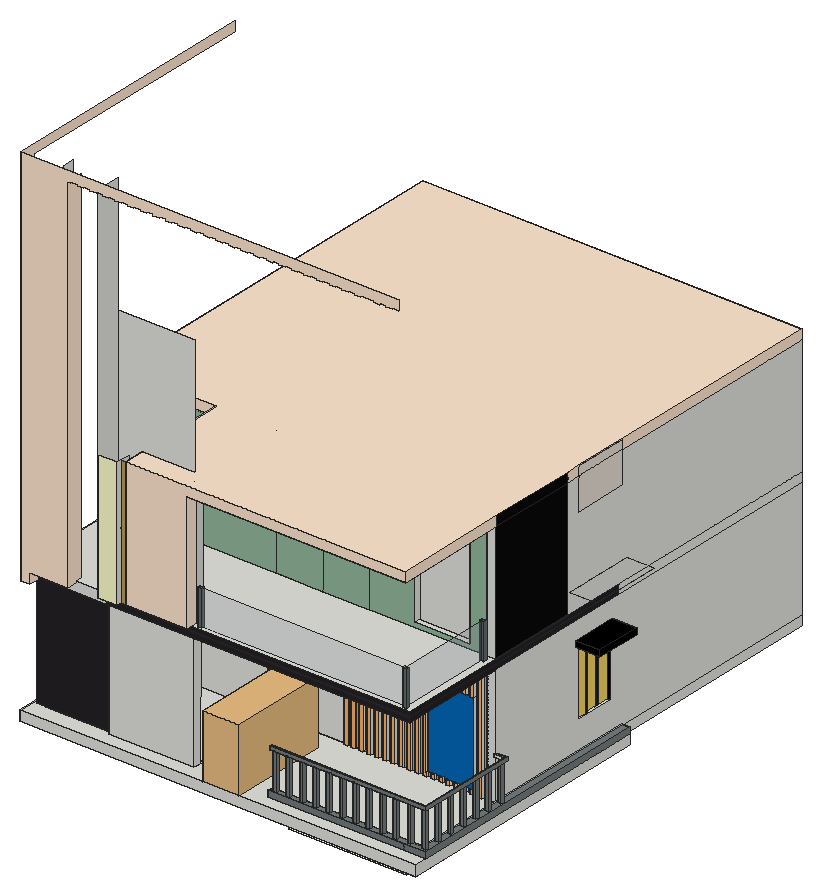
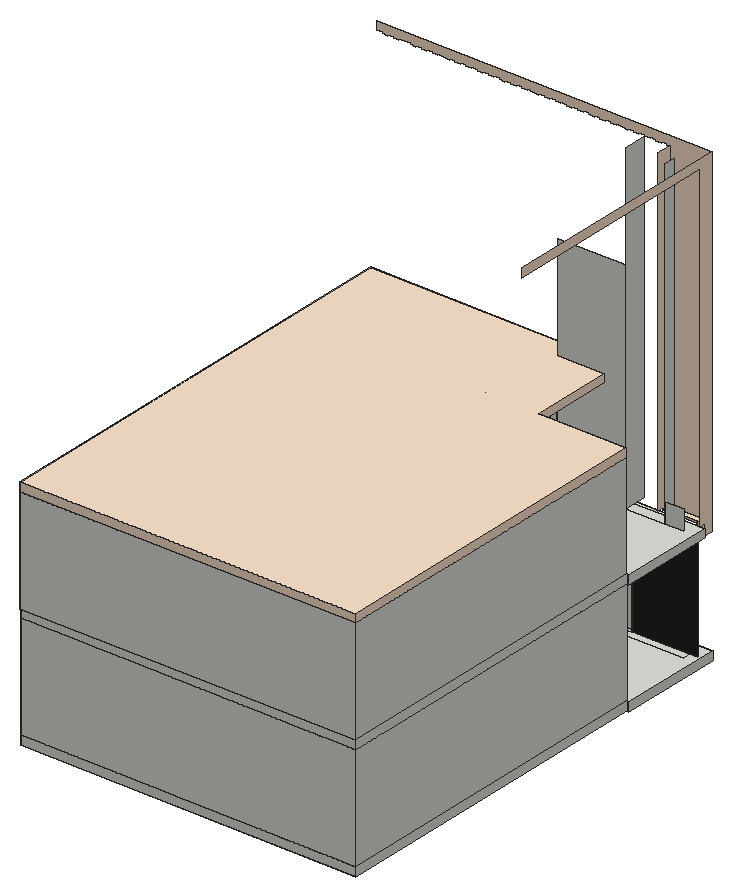
# SketchUp Ruby script. Lengths in inches.
U = 1.inch
M = Sketchup.active_model
def pt(a) = Geom::Point3d.new(a.map { |v| v * U })
def face(e, loops, mat)
  f = e.add_face(loops[0].map { |a| pt(a) })
  loops[1..].each { |l| e.add_face(l.map { |a| pt(a) }).erase! }
  f.material = f.back_material = mat if mat
  f
end
# faces: each face lists its corners as indices into pts; further lists are holes
def faces(e, pts, list, mat = nil) = list.each { |f| face(e, (f[0].is_a?(Array) ? f : [f]).map { |l| l.map { |i| pts[i] } }, mat) }
# xy, xz, yz: faces in a plane at the given z, y or x. An outline is a flat list of corners, or four numbers for a rectangle; further outlines are holes
def ring(l) = l.size == 4 ? [[l[0], l[1]], [l[2], l[1]], [l[2], l[3]], [l[0], l[3]]] : l.each_slice(2).to_a
def flat(e, list, mat, &to3) = list.each { |f| face(e, (f[0].is_a?(Array) ? f : [f]).map { |l| ring(l).map { |u, v| to3.(u, v) } }, mat) }
def xy(e, z, list, mat = nil) = flat(e, list, mat) { |x, y| [x, y, z] }
def xz(e, y, list, mat = nil) = flat(e, list, mat) { |x, z| [x, y, z] }
def yz(e, x, list, mat = nil) = flat(e, list, mat) { |y, z| [x, y, z] }
def lines(e, pts, list) = list.each { |a, b| e.add_line(pt(pts[a]), pt(pts[b])) }
# prism: a flat outline (further loops are holes) pulled along v
def prism(e, loops, v, mat = nil)
  f = face(e, loops, mat); d = Geom::Vector3d.new(v.map { |x| x * U })
  f.pushpull(f.normal.samedirection?(d) ? d.length : -d.length)
end
def box(e, o, s, mat = nil) = prism(e, [[o, [o[0] + s[0], o[1], o[2]], [o[0] + s[0], o[1] + s[1], o[2]], [o[0], o[1] + s[1], o[2]]]], [0, 0, s[2]], mat)
def at(x, y, z, deg = 0) = Geom::Transformation.translation(pt([x, y, z])) * Geom::Transformation.rotation(ORIGIN, Z_AXIS, deg.degrees)
def axes(o, x, y, z) = Geom::Transformation.new([*x, 0, *y, 0, *z, 0, *pt(o).to_a, 1])
def part(name) = M.definitions.add(name)
# library, detail: a bought-in or finely detailed component or shape, given as its bounding box
def library(name, o, s) = part(name).tap { |d| box(d.entities, o, s) }
def detail(e, o, s) = box(e.add_group.entities, o, s)
def put(e, d, t, mat = nil) = e.add_instance(d, t).tap { |i| i.material = mat if mat }
def group(e, t, mat = nil) = e.add_group.tap { |g| g.transformation = t; g.material = mat if mat }.entities
root = M.entities
M.materials.add("C01_Vanilla_Cream").color = [255, 230, 206]
M.materials.add("C03_Honey_Glow").color = [255, 178, 101]
M.materials.add("C04_Amber_Sunshine").color = [255, 152, 49]
M.materials.add("C05_Golden_Blaze").color = [255, 123, 0]
M.materials.add("E01_Mint_Frost").color = [255, 255, 204]
M.materials.add("Glass_Basic_01").color = [161, 173, 186]
M.materials["Glass_Basic_01"].alpha = 0.25
M.materials.add("Glass_Mirror_01").color = [4, 105, 185]
M.materials.add("Glass_Mirror_2").color = [185, 158, 90]
M.materials.add("Glass_Mirror_3").color = [244, 212, 100]
M.materials.add("Glass_Mirror_4").color = [147, 185, 156]
M.materials.add("GreyOffset").color = [97, 108, 109]
M.materials.add("M08_Obsidian_Black1").color = [30, 30, 30]
M.materials.add("M09_Shadow_Night").color = [0, 0, 0]
M.materials.add("Marble_01_1K").color = [230, 221, 211]
M.materials.add("Marble_07_1K").color = [36, 34, 36]
M.materials.add("Metal_32_1K").color = [117, 124, 125]
M.materials.add("NERO MARQUINA 02").color = [10, 10, 10]
M.materials.add("[Color_000]").color = [255, 255, 255]
c1 = part("Group\#12")
xy(c1.entities,36,[[0,0,3.82,2.79]],"Metal_32_1K")
xz(c1.entities,0,[[0,0,3.82,36]],"Metal_32_1K")
xz(c1.entities,2.79,[[0,0,3.82,36]],"Metal_32_1K")
yz(c1.entities,0,[[0,0,2.79,36]],"Metal_32_1K")
yz(c1.entities,3.82,[[0,0,2.79,36]],"Metal_32_1K")
c2 = part("Group\#11")
xy(c2.entities,36,[[0,0,3.82,2.79]],"Metal_32_1K")
xz(c2.entities,0,[[0,0,3.82,36]],"Metal_32_1K")
xz(c2.entities,2.79,[[0,0,3.82,36]],"Metal_32_1K")
yz(c2.entities,0,[[0,0,2.79,36]],"Metal_32_1K")
yz(c2.entities,3.82,[[0,0,2.79,36]],"Metal_32_1K")
c3 = library("Group_2",[-1.28,-0.39,0],[21.22,20.51,48.44])
xy(root,97.49,[[307.1875,182.1,366.58,186.51],[366.83,182.1,426.21,186.22]],"[Color_000]")
xy(root,120,[[60.23,165,180,171],[222,171,287.05,179.92],[222,179.92,287.05,180],[222,180,287.05,204.3],[435.75,196.73,444.75,197.01,444,220.51,444,273,435,273,435,220.22]])
xy(root,130,[[135.41,168,222,171],[69,171,222,179.92]])
xy(root,249.85,[[60,151,69,161]],"C01_Vanilla_Cream")
xy(root,259.85,[[135.55,154,155.45,168],[89.98,168,135.55,180]])
xy(root,259.85,[[69,151,107.56,161]],"C01_Vanilla_Cream")
xz(root,151,[[60,249.85,69,249.85,69,259.85,107.56,259.85,107.56,628.54,111.09,628.54,111.09,629.54,117.48,629.54,117.48,628.54,123.87,628.54,123.87,629.54,130.25,629.54,130.25,628.54,136.64,628.54,136.64,629.54,143.03,629.54,143.03,628.54,149.41,628.54,149.41,629.54,155.8,629.54,155.8,628.54,162.1875,628.54,162.1875,629.54,168.57,629.54,168.57,628.54,174.96,628.54,174.96,629.54,181.35,629.54,181.35,628.54,187.73,628.54,187.73,629.54,194.12,629.54,194.12,628.54,200.51,628.54,200.51,629.54,206.89,629.54,206.89,628.54,213.28,628.54,213.28,629.54,219.67,629.54,219.67,628.54,226.05,628.54,226.05,629.54,232.4375,629.54,232.4375,628.54,238.83,628.54,238.83,629.54,245.21,629.54,245.21,628.54,251.6,628.54,251.6,629.54,257.98,629.54,257.98,628.54,264.37,628.54,264.37,629.54,270.76,629.54,270.76,628.54,277.14,628.54,277.14,629.54,283.53,629.54,283.53,628.54,289.92,628.54,289.92,629.54,296.3,629.54,296.3,628.54,302.69,628.54,302.69,629.54,309.08,629.54,309.08,628.54,315.46,628.54,315.46,629.54,321.85,629.54,321.85,628.54,328.24,628.54,328.24,629.54,334.625,629.54,334.625,628.54,341.01,628.54,341.01,629.54,347.4,629.54,347.4,628.54,353.78,628.54,353.78,629.54,360.17,629.54,360.17,628.54,366.56,628.54,366.56,629.54,372.94,629.54,372.94,628.54,379.33,628.54,379.33,629.54,385.72,629.54,385.72,628.54,392.1,628.54,392.1,629.54,398.49,629.54,398.49,628.54,404.88,628.54,404.88,629.54,417.65,629.54,417.65,628.54,424.04,628.54,424.04,629.54,430.42,629.54,430.42,628.54,436.81,628.54,436.81,629.54,443.2,629.54,443.2,639.54,60,639.54]],"C01_Vanilla_Cream")
xz(root,154,[[135.55,259.85,155.45,389.69]],"E01_Mint_Frost")
xz(root,159,[[155.45,259.85,160.13,389.69]],"Glass_Mirror_2")
xz(root,161,[[60,249.85,69,261.88],[69,259.85,107.56,261.88]],"C01_Vanilla_Cream")
xz(root,168,[[135.41,130,222,249.85]])
xz(root,168.1,[[230.8,259.85,434.6,295.85]],"Glass_Basic_01")
xz(root,171,[[60,130,135.41,249.85]],"Marble_07_1K")
xz(root,180,[[69,259.85,89.98,282.89],[135.55,259.85,213,509.54]])
yz(root,60,[[151,249.85,151,639.54,422.07,639.54,422.07,629.54,168,629.54,168,261.88,161,261.88,161,249.85]],"C01_Vanilla_Cream")
yz(root,69,[[151,249.85,161,259.85]],"C01_Vanilla_Cream")
yz(root,89.98,[[168,259.85,180,629.54]])
yz(root,107.56,[[151,259.85,161,259.85,161,261.88,168,261.88,168,628.54,151,628.54]],"C01_Vanilla_Cream")
yz(root,135.41,[[168,130,171,249.85]])
yz(root,135.55,[[154,259.85,180,629.54]])
yz(root,155.45,[[154,259.85,159,389.69],[159,259.85,168,389.69]])
yz(root,222,[[168,130,175.46,130,176.59,249.8,176.59,249.85,168,249.85]])
yz(root,436.72,[[169.55,259.85,264.51,295.85]],"Glass_Basic_01")
p = [[222.23,171,379.69],[222.23,171,259.85],[221.39,180,259.85],[221.39,180,379.69],[222,168,249.85],[222,168,389.69],
  [444,363.42,259.85],[444,273.3,259.85],[213,180,259.85]]
faces(root,p,[[0,1,2,3]])
lines(root,p,[[4,5],[6,7],[8,2]])
g1 = group(root,at(60,273,120))
xy(g1,0,[[-3,-119.23,-3,0,0,0,0,387,384,387,384,152.46,397.91,152.46,397.91,-119.23]])
xy(g1,10,[[-3,-119.23,397.91,-119.23,397.91,-105.79,237.85,-105.79,237.85,-100,389.74,-100,389.74,152.46,384,152.46,384,387,0,387,0,0,-3,0],[237.85,-105.79,397.91,-105.79,397.91,152.46,389.74,152.46,389.74,-100,237.85,-100]])
xy(g1,16,[[237.85,-105.79,397.91,-105.79,397.91,152.46,389.74,152.46,389.74,-100,237.85,-100]],"Metal_32_1K")
xy(g1,52,[[237.68,-103.375,237.68,-101.59,378.28,-101.59,378.28,-101.48,393.9,-101.48,393.9,-2.71,384,-2.71,384,0,395.84,0,395.84,-103.375]])
xy(g1,55,[[237.68,-103.375,395.84,-103.375,395.84,0,384,0,384,-2.71,393.9,-2.71,393.9,-101.48,378.28,-101.48,378.28,-101.59,237.68,-101.59]],"Metal_32_1K")
xz(g1,-119.23,[[-3,0,397.91,10]])
xz(g1,-105.79,[[237.85,10,375,16],[375,10,397.91,16]],"Metal_32_1K")
xz(g1,-103.375,[[237.68,52,395.84,55]],"Metal_32_1K")
xz(g1,-101.59,[[237.68,52,378.28,55]],"Metal_32_1K")
xz(g1,-101.48,[[378.28,52,393.9,55]])
xz(g1,-100,[[237.85,10,375,16],[375,10,389.74,16]])
xz(g1,-2.71,[[384,52,393.9,55]])
xz(g1,0,[[-3,0,0,10],[384,52,395.84,55]])
xz(g1,152.46,[[384,0,397.91,9.85],[384,9.85,397.91,10],[389.74,10,397.91,16]])
xz(g1,387,[[0,0,384,10]])
yz(g1,-3,[[-119.23,0,0,10]])
yz(g1,0,[[0,0,387,10]])
yz(g1,237.68,[[-103.375,52,-101.59,55]],"Metal_32_1K")
yz(g1,237.85,[[-105.79,10,-100,16]],"Metal_32_1K")
yz(g1,378.28,[[-101.59,52,-101.48,55]])
yz(g1,384,[[152.46,0,387,10],[-2.71,52,0,55]])
yz(g1,389.74,[[-100,10,152.46,16]])
yz(g1,393.9,[[-101.48,52,-2.71,55]])
yz(g1,395.84,[[-103.375,52,0,55]],"Metal_32_1K")
yz(g1,397.91,[[-119.23,0,152.46,10]])
yz(g1,397.91,[[-105.79,10,152.46,16]],"Metal_32_1K")
put(g1,c1,at(322.36,-104.375,16))
put(g1,c1,at(241.23,-104.375,16))
put(g1,c1,at(281.8,-104.375,16))
put(g1,c1,at(254.75,-104.375,16))
put(g1,c1,at(268.27,-104.375,16))
put(g1,c1,at(295.32,-104.375,16))
put(g1,c1,at(308.84,-104.375,16))
put(g1,c1,at(362.93,-104.375,16))
put(g1,c1,at(349.41,-104.375,16))
put(g1,c2,at(376.45,-102.79,16))
put(g1,c1,at(335.89,-104.375,16))
put(g1,c2,at(391.57,-102.79,16))
put(g1,c2,at(391.57,-86.92,16))
put(g1,c2,at(391.57,-71.0625,16))
put(g1,c2,at(391.57,-55.2,16))
put(g1,c2,at(391.57,-39.34,16))
put(g1,c2,at(391.57,-23.48,16))
put(g1,c2,at(391.57,-7.62,16))
g2 = group(root,at(60,273,129.85))
xy(g2,0,[[153,0,375,0,375,378,9,378,9,6,153,6]])
xy(g2,0.15,[[255,-2,259.01,0],[263.03,-2,267.04,0],[271.06,-2,275.07,0],[279.09,-2,283.1,0],[287.11,-2,291.13,0],
  [295.14,-2,299.16,0],[303.17,-2,307.19,0],[311.2,-2,315.21,0],[319.23,-2,323.24,0],[327.26,-2,331.27,0],
  [335.28,-2,339.3,0],[343.3125,-2,347.33,0],[351.34,-2,355.36,0],[359.37,-2,363.38,0],[367.4,-2,371.41,0]])
xy(g2,4.55,[[315,-2,315.21,0],[319.23,-2,323.24,-2,323.24,-0.34,319.23,-0.17],[327.26,-2,331.27,-2,331.27,-0.67,327.26,-0.5],[335.28,-2,339.3,-2,339.3,-1.01,335.28,-0.84],[343.3125,-2,347.33,-2,347.33,-1.34,343.3125,-1.18],
  [351.34,-2,355.36,-2,355.36,-1.68,351.34,-1.51],[359.37,-2,363,-2,359.37,-1.85],[363,-2,363,0,359.37,0,359.37,-1.85],[359.37,-1.85,359.37,0,355.36,0,355.36,-1.68],[355.36,-1.68,355.36,0,351.34,0,351.34,-1.51],
  [351.34,-1.51,351.34,0,347.33,0,347.33,-1.34],[347.33,-1.34,347.33,0,343.3125,0,343.3125,-1.18],[343.3125,-1.18,343.3125,0,339.3,0,339.3,-1.01],[339.3,-1.01,339.3,0,335.28,0,335.28,-0.84],[335.28,-0.84,335.28,0,331.27,0,331.27,-0.67],
  [331.27,-0.67,331.27,0,327.26,0,327.26,-0.5],[327.26,-0.5,327.26,0,323.24,0,323.24,-0.34],[323.24,-0.34,323.24,0,319.23,0,319.23,-0.17],[319.23,-0.17,319.23,0,315.21,0],[315.21,0,363,22.25]])
xy(g2,21.14,[[376.51,129.93,380.31,133.17]])
xy(g2,28.66,[[376.11,115.5,381.52,117.99]])
xy(g2,29.18,[[375,103.49,384,145.28]])
xy(g2,88.55,[[315,-2,315.21,0],[319.23,-2,319.23,-0.17,323.24,-0.34,323.24,-2],[327.26,-2,327.26,-0.5,331.27,-0.67,331.27,-2],[335.28,-2,335.28,-0.84,339.3,-1.01,339.3,-2],[343.3125,-2,343.3125,-1.18,347.33,-1.34,347.33,-2],
  [351.34,-2,351.34,-1.51,355.36,-1.68,355.36,-2],[359.37,-2,359.37,-1.85,363,-2],[363,-2,359.37,-1.85,359.37,0,363,0],[359.37,-1.85,355.36,-1.68,355.36,0,359.37,0],[355.36,-1.68,351.34,-1.51,351.34,0,355.36,0],
  [351.34,-1.51,347.33,-1.34,347.33,0,351.34,0],[347.33,-1.34,343.3125,-1.18,343.3125,0,347.33,0],[343.3125,-1.18,339.3,-1.01,339.3,0,343.3125,0],[339.3,-1.01,335.28,-0.84,335.28,0,339.3,0],[335.28,-0.84,331.27,-0.67,331.27,0,335.28,0],
  [331.27,-0.67,327.26,-0.5,327.26,0,331.27,0],[327.26,-0.5,323.24,-0.34,323.24,0,327.26,0],[323.24,-0.34,319.23,-0.17,319.23,0,323.24,0],[319.23,-0.17,315.21,0,319.23,0],[315.21,0,363,22.25]])
xy(g2,94.04,[[375,103.49,375,145.28,380.31,145.28,380.31,133.17,376.51,133.17,376.51,129.93,380.31,129.93,380.31,117.99,376.11,117.99,376.11,115.5,381.52,115.5,381.52,103.49],[381.52,103.49,381.52,117.99,380.31,117.99,380.31,145.28,384,145.28,384,103.49]])
xy(g2,96.89,[[384,100.07,409.01,146.84]],"M09_Shadow_Night")
xy(g2,103.11,[[384,100.07,409.01,146.84]],"M09_Shadow_Night")
xy(g2,120,[[255,-2,259.01,0],[263.03,-2,267.04,0],[271.06,-2,275.07,0],[279.09,-2,283.1,0],[287.11,-2,291.13,0],
  [295.14,-2,299.16,0],[303.17,-2,307.19,0],[311.2,-2,315.21,0],[319.23,-2,323.24,0],[327.26,-2,331.27,0],
  [335.28,-2,339.3,0],[343.3125,-2,347.33,0],[351.34,-2,355.36,0],[359.37,-2,363.38,0],[367.4,-2,371.41,0],
  [0,0,153,0,153,6,9,6,9,378,375,378,375,0,384,0,384,387,0,387]])
xz(g2,-2,[[231,0.15,235.01,120],[239,0.15,243.01,120],[247,0.15,251.01,120],[255,0.15,259.01,120],[263.03,0.15,267.04,120],
  [271.06,0.15,275.07,120],[279.09,0.15,283.1,120],[287.11,0.15,291.13,120],[295.14,0.15,299.16,120],[303.17,0.15,307.19,120],
  [311.2,0.15,315.21,0.15,315.21,4.55,315,4.55,315,88.55,315.21,88.55,315.21,120,311.2,120],[319.23,0.15,323.24,4.55],[327.26,0.15,331.27,4.55],[335.28,0.15,339.3,4.55],[343.3125,0.15,347.33,4.55],
  [351.34,0.15,355.36,4.55],[359.37,0.15,363.38,0.15,363.38,88.55,363,88.55,363,4.55,359.37,4.55],[367.4,0.15,371.41,120],[319.23,88.55,323.24,120],[327.26,88.55,331.27,120],
  [335.28,88.55,339.3,120],[343.3125,88.55,347.33,120],[351.34,88.55,355.36,120],[359.37,88.55,363.38,120]],"C03_Honey_Glow")
xz(g2,0,[[9,0,9,120,0,120,0,0.15],[9,0,153,120],[153,0,375,0.15],[375,0,384,0,384,120,375.43,120,375.43,0.15,375,0.15],[153,0.15,231,120],
  [231,0.15,235.01,120],[239,0.15,243.01,120],[247,0.15,251.01,120],[319.23,0.15,323.24,4.55],[327.26,0.15,331.27,4.55],
  [335.28,0.15,339.3,4.55],[343.3125,0.15,347.33,4.55],[351.34,0.15,355.36,4.55],[359.37,0.15,363.38,0.15,363.38,120,359.37,120,359.37,88.55,363,88.55,363,4.55,359.37,4.55],[375,0.15,375.43,120],
  [315,4.55,315.21,88.55],[315.21,4.55,363,88.55],[319.23,88.55,323.24,120],[327.26,88.55,331.27,120],[335.28,88.55,339.3,120],
  [343.3125,88.55,347.33,120],[351.34,88.55,355.36,120]])
xz(g2,0,[[235.01,0.15,239,120],[243.01,0.15,247,120],[251.01,0.15,255,120],[259.01,0.15,263.03,120],[267.04,0.15,271.06,120],
  [275.07,0.15,279.09,120],[283.1,0.15,287.11,120],[291.13,0.15,295.14,120],[299.16,0.15,303.17,120],[307.19,0.15,311.2,120],
  [315.21,0.15,319.23,4.55],[323.24,0.15,327.26,4.55],[331.27,0.15,335.28,4.55],[339.3,0.15,343.3125,4.55],[347.33,0.15,351.34,4.55],
  [355.36,0.15,359.37,4.55],[363.38,0.15,367.4,120],[371.41,0.15,375,120],[315.21,88.55,319.23,120],[323.24,88.55,327.26,120],
  [331.27,88.55,335.28,120],[339.3,88.55,343.3125,120],[347.33,88.55,351.34,120],[355.36,88.55,359.37,120]],"C04_Amber_Sunshine")
xz(g2,6,[[9,0,153,120]])
xz(g2,22.25,[[315.21,4.55,363,88.55]])
xz(g2,100.07,[[384,96.89,409.01,103.11]],"M09_Shadow_Night")
xz(g2,103.49,[[375,29.18,381.52,94.04]])
xz(g2,103.49,[[381.52,29.18,384,94.04]],"M09_Shadow_Night")
xz(g2,115.5,[[376.11,28.66,381.52,94.04]])
xz(g2,117.99,[[376.11,28.66,381.52,94.04]])
xz(g2,129.93,[[376.51,21.14,380.31,94.04]])
xz(g2,133.17,[[376.51,21.14,380.31,94.04]])
xz(g2,145.28,[[375,29.18,380.31,94.04]])
xz(g2,145.28,[[380.31,29.18,384,94.04]],"M09_Shadow_Night")
xz(g2,146.84,[[384,96.89,409.01,103.11]],"M09_Shadow_Night")
xz(g2,378,[[9,0,375,120]])
xz(g2,387,[[0,0,384,120]])
yz(g2,0,[[387,0,0,0.15,0,120,387,120]])
yz(g2,9,[[6,0,378,120]])
yz(g2,153,[[0,0,6,120]])
yz(g2,231,[[-2,0.15,0,120]])
yz(g2,239,[[-2,0.15,0,120]])
yz(g2,247,[[-2,0.15,0,120]])
yz(g2,255,[[-2,0.15,0,120]])
yz(g2,259.01,[[-2,0.15,0,120]])
yz(g2,263.03,[[-2,0.15,0,120]])
yz(g2,267.04,[[-2,0.15,0,120]])
yz(g2,271.06,[[-2,0.15,0,120]])
yz(g2,275.07,[[-2,0.15,0,120]])
yz(g2,279.09,[[-2,0.15,0,120]])
yz(g2,283.1,[[-2,0.15,0,120]])
yz(g2,287.11,[[-2,0.15,0,120]])
yz(g2,291.13,[[-2,0.15,0,120]])
yz(g2,295.14,[[-2,0.15,0,120]])
yz(g2,299.16,[[-2,0.15,0,120]])
yz(g2,303.17,[[-2,0.15,0,120]])
yz(g2,307.19,[[-2,0.15,0,120]])
yz(g2,311.2,[[-2,0.15,0,120]])
yz(g2,315,[[-2,4.55,0,88.55]])
yz(g2,315.21,[[-2,0.15,0,4.55],[0,4.55,22.25,88.55],[-2,88.55,0,120]])
yz(g2,319.23,[[-2,0.15,0,4.55],[-2,88.55,0,120]])
yz(g2,323.24,[[-2,0.15,0,4.55],[-2,88.55,0,120]])
yz(g2,327.26,[[-2,0.15,0,4.55],[-2,88.55,0,120]])
yz(g2,331.27,[[-2,0.15,0,4.55],[-2,88.55,0,120]])
yz(g2,335.28,[[-2,0.15,0,4.55],[-2,88.55,0,120]])
yz(g2,339.3,[[-2,0.15,0,4.55],[-2,88.55,0,120]])
yz(g2,343.3125,[[-2,0.15,0,4.55],[-2,88.55,0,120]])
yz(g2,347.33,[[-2,0.15,0,4.55],[-2,88.55,0,120]])
yz(g2,351.34,[[-2,0.15,0,4.55],[-2,88.55,0,120]])
yz(g2,355.36,[[-2,0.15,0,4.55],[-2,88.55,0,120]])
yz(g2,359.37,[[-2,0.15,0,4.55],[-2,88.55,0,120]])
yz(g2,363,[[-2,4.55,0,88.55],[0,4.55,22.25,88.55]])
yz(g2,363.38,[[-2,0.15,0,88.55],[-2,88.55,0,120]])
yz(g2,367.4,[[-2,0.15,0,120]])
yz(g2,371.41,[[-2,0.15,0,120]])
yz(g2,375,[[[0,0,378,120],[103.49,29.18,145.28,94.04]]])
yz(g2,376.11,[[115.5,28.66,117.99,94.04]])
yz(g2,376.51,[[129.93,21.14,133.17,94.04]])
yz(g2,380.31,[[117.99,29.18,129.93,94.04],[133.17,29.18,145.28,94.04]],"Glass_Mirror_3")
yz(g2,380.31,[[129.93,21.14,133.17,94.04]],"M08_Obsidian_Black1")
yz(g2,381.52,[[103.49,29.18,115.5,94.04]],"Glass_Mirror_3")
yz(g2,381.52,[[115.5,28.66,117.99,94.04]],"M08_Obsidian_Black1")
yz(g2,384,[[[0,0,387,120],[103.49,29.18,145.28,94.04],[100.07,96.89,146.84,103.11]]])
yz(g2,409.01,[[100.07,96.89,146.84,103.11]],"M09_Shadow_Night")
p = [[315.21,0,88.55],[315.21,0,4.55],[319.23,-0.17,4.55],[323.24,-0.34,4.55],[327.26,-0.5,4.55],[331.27,-0.67,4.55],
  [335.28,-0.84,4.55],[339.3,-1.01,4.55],[343.3125,-1.18,4.55],[347.33,-1.34,4.55],[351.34,-1.51,4.55],[355.36,-1.68,4.55],
  [359.37,-1.85,4.55],[363,-2,4.55],[363,-2,88.55],[359.37,-1.85,88.55],[355.36,-1.68,88.55],[351.34,-1.51,88.55],
  [347.33,-1.34,88.55],[343.3125,-1.18,88.55],[339.3,-1.01,88.55],[335.28,-0.84,88.55],[331.27,-0.67,88.55],[327.26,-0.5,88.55],
  [323.24,-0.34,88.55],[319.23,-0.17,88.55],[375.43,0,0.15],[376.1,0,0.15],[251.01,0,0.15],[251.01,-2,0.15],
  [243.01,0,0.15],[243.01,-2,0.15],[235.01,0,0.15],[235.01,-2,0.15]]
faces(g2,p,[[0,1,2,3,4,5,6,7,8,9,10,11,12,13,14,15,16,17,18,19,20,21,22,23,24,25]],"Glass_Mirror_01")
lines(g2,p,[[26,27],[28,29],[30,31],[32,33]])
put(root,c3,axes([244.4,251.01,130],[1.75,0,0],[0,-4.83227,0],[0,0,1.34]))
g3 = group(root,at(60,273,249.85))
xy(g3,0,[[-3,-109,-3,0,0,0,0,387,384,387,384,-109]])
xy(g3,5.98,[[75.55,-109,76.05,-108.5],[76.05,-109,384,-108.5],[383.65,-108.5,384,155.66]])
xy(g3,10,[[-3,-109,384,-109,384,387,0,387,0,0,-3,0]])
xz(g3,-109,[[-3,0,75.55,0,75.55,5.04,76.05,5.04,76.05,5.98,75.55,5.98,75.55,10,-3,10]])
xz(g3,-109,[[75.55,0,384,0,384,4.99,76.05,5.04,75.55,5.04],[75.55,5.98,384,10]],"Marble_07_1K")
xz(g3,-108.5,[[383.65,4.99,383.65,5.98,76.05,5.98,76.05,5.04]])
xz(g3,0,[[-3,0,0,10]])
xz(g3,155.66,[[383.65,4.98,384,5.98]])
xz(g3,387,[[0,0,384,10]])
yz(g3,-3,[[-109,0,0,10]])
yz(g3,0,[[0,0,387,10]])
yz(g3,76.05,[[-109,5.04,-108.5,5.98]])
yz(g3,383.65,[[155.66,4.98,155.66,5.98,-108.5,5.98,-108.5,4.99]])
yz(g3,384,[[155.66,0,387,10]])
yz(g3,384,[[-109,0,155.66,0,155.66,4.98,-108.5,4.99,-109,4.99],[-109,5.98,155.66,10]],"Marble_07_1K")
p = [[76.05,-108.5,5.04],[76.05,-109,5.04],[384,-109,4.99],[384,-108.5,4.99],[383.65,-108.5,4.99],[384,155.66,4.98],
  [383.65,155.66,4.98]]
faces(g3,p,[[0,1,2,3,4],[3,5,6,4]])
g4 = group(root,at(60,273.3,259.69))
xy(g4,0,[[9,6,375,378]])
xy(g4,4.95,[[301.4,0,357.2,12.97]])
xy(g4,102.65,[[301.4,0,357.2,12.97]])
xy(g4,120,[[0,0,375,0,375,6,9,6,9,378,375,378,375,0,384,0,384,387,0,387]])
xz(g4,-0.42,[[174.25,61.12,174.61,61.12,174.61,102.58]])
xz(g4,-0.42,[[162,0.29,208.81,61.12],[208.81,0.29,255.62,61.12],[162,61.12,174.25,61.12,174.61,102.58,162,102.58]],"Glass_Mirror_4")
xz(g4,0,[[9,0,9,120,0,120,0,0.15],[375,0,384,120]])
xz(g4,0,[[9,0,375,0,375,120,301.4,120,301.4,102.65,357.2,102.65,357.2,4.95,301.4,4.95,301.4,120,9,120]],"Glass_Mirror_4")
xz(g4,6,[[9,0,153,120],[153,0,375,120]])
xz(g4,12.97,[[301.4,4.95,357.2,102.65]])
xz(g4,378,[[9,0,375,120]])
xz(g4,387,[[0,0,384,120]])
yz(g4,0,[[387,0,0,0.15,0,120,387,120]])
yz(g4,9,[[6,0,378,120]])
yz(g4,301.4,[[0,4.95,12.97,102.65]])
yz(g4,357.2,[[0,4.95,12.97,102.65]])
yz(g4,375,[[0,0,6,120],[6,0,378,120]])
yz(g4,384,[[0,0,387,0,387,120,159.34,120,159.34,88.12,105.01,88.12,105.01,120,90.12,120,90.12,0.15,0,0.15]])
yz(g4,384,[[105.01,88.12,159.34,120]],"Marble_01_1K")
yz(g4,384,[[0,0.15,90.12,120]],"NERO MARQUINA 02")
p = [[174.61,-0.42,102.58],[174.61,-0.42,61.12],[301.4,0,61.12],[301.4,0,102.58],[403.5,165.34,20.0625],[384,165.34,20.0625],
  [384,92.68,20.0625],[411.82,92.68,20.0625],[411.82,165.34,20.0625],[406.1,165.34,20.0625],[299.84,-0.42,102.58],[301.4,0,102.65],
  [255.62,-0.42,0.2],[255.62,-0.42,0.29],[208.81,-0.42,0.29],[208.81,-0.42,0.2],[255.68,-0.42,0.29]]
faces(g4,p,[[0,1,2,3]],"Glass_Mirror_4")
lines(g4,p,[[4,5],[5,6],[6,7],[7,8],[8,9],[10,11],[0,10],[12,13],[14,15],[13,16]])
g5 = group(root,at(226.57,166.66,259.85))
xy(g5,0,[[0,0,4.24,2.89]])
xy(g5,36,[[0,0,4.24,2.89]],"GreyOffset")
xz(g5,0,[[0,0,4.24,36]],"GreyOffset")
xz(g5,2.89,[[0,0,4.24,36]],"GreyOffset")
yz(g5,0,[[0,0,2.89,36]],"GreyOffset")
yz(g5,4.24,[[0,0,2.89,36]],"GreyOffset")
g6 = group(root,at(434.6,166.66,259.85))
xy(g6,0,[[0,0,4.24,2.89]])
xy(g6,36,[[0,0,4.24,2.89]],"GreyOffset")
xz(g6,0,[[0,0,4.24,36]],"GreyOffset")
xz(g6,2.89,[[0,0,4.24,36]],"GreyOffset")
yz(g6,0,[[0,0,2.89,36]])
yz(g6,4.24,[[0,0,2.89,36]],"GreyOffset")
g7 = group(root,at(434.6,264.51,259.85))
xy(g7,0,[[0,0,4.24,2.89]])
xy(g7,36,[[0,0,4.24,2.89]],"GreyOffset")
xz(g7,0,[[0,0,4.24,36]],"GreyOffset")
xz(g7,2.89,[[0,0,4.24,36]],"GreyOffset")
yz(g7,0,[[0,0,2.89,36]],"GreyOffset")
yz(g7,4.24,[[0,0,2.89,36]],"GreyOffset")
g8 = group(root,at(60,366.3,379.69),"C01_Vanilla_Cream")
xy(g8,-119.85,[[100.13,-207.3,162.23,-195.3]])
xy(g8,0,[[162.23,-207.3,384,-195.3],[100.13,-195.3,100.13,-93,0,-93,0,294,384,294,384,-93,162.23,-93,162.23,-195.3],[162.23,-195.3,165.93,-93],[169.625,-195.3,173.32,-93],[177.02,-195.3,180.71,-93],
  [184.41,-195.3,188.11,-93],[191.8,-195.3,195.5,-93],[199.19,-195.3,202.89,-93],[206.59,-195.3,210.28,-93],[213.98,-195.3,217.68,-93],
  [221.37,-195.3,225.07,-93],[228.76,-195.3,232.46,-93],[236.16,-195.3,239.85,-93],[243.55,-195.3,247.24,-93],[250.94,-195.3,254.64,-93],
  [258.33,-195.3,262.03,-93],[265.72,-195.3,269.42,-93],[273.12,-195.3,276.8125,-93],[280.51,-195.3,284.21,-93],[287.9,-195.3,291.6,-93],
  [295.29,-195.3,298.99,-93],[302.6875,-195.3,306.38,-93],[310.08,-195.3,313.77,-93],[317.47,-195.3,321.17,-93],[324.86,-195.3,328.56,-93],
  [332.25,-195.3,335.95,-93],[347.04,-195.3,350.74,-93],[354.43,-195.3,358.13,-93],[361.82,-195.3,365.52,-93],[369.22,-195.3,372.91,-93],
  [376.61,-195.3,380.3,-93]])
xy(g8,0,[[339.65,-195.3,343.34,-93]],"C01_Vanilla_Cream")
xy(g8,0,[[165.93,-195.3,169.625,-93],[173.32,-195.3,177.02,-93],[180.71,-195.3,184.41,-93],[188.11,-195.3,191.8,-93],[195.5,-195.3,199.19,-93],
  [202.89,-195.3,206.59,-93],[210.28,-195.3,213.98,-93],[217.68,-195.3,221.37,-93],[225.07,-195.3,228.76,-93],[232.46,-195.3,236.16,-93],
  [239.85,-195.3,243.55,-93],[247.24,-195.3,250.94,-93],[254.64,-195.3,258.33,-93],[262.03,-195.3,265.72,-93],[269.42,-195.3,273.12,-93],
  [276.8125,-195.3,280.51,-93],[284.21,-195.3,287.9,-93],[291.6,-195.3,295.29,-93],[298.99,-195.3,302.6875,-93],[306.38,-195.3,310.08,-93],
  [313.77,-195.3,317.47,-93],[321.17,-195.3,324.86,-93],[328.56,-195.3,332.25,-93],[335.95,-195.3,339.65,-93],[343.34,-195.3,347.04,-93],
  [350.74,-195.3,354.43,-93],[358.13,-195.3,361.82,-93],[365.52,-195.3,369.22,-93],[372.91,-195.3,376.61,-93],[380.3,-195.3,384,-93]],"C05_Golden_Blaze")
xy(g8,10,[[100.13,-207.3,384,-207.3,384,294,0,294,0,-93,100.13,-93]],"C01_Vanilla_Cream")
xz(g8,-207.3,[[100.13,-119.85,162.23,-119.85,162.23,0,384,0,384,10,100.13,10]],"C01_Vanilla_Cream")
xz(g8,-195.3,[[100.13,-119.85,101.09,0],[101.09,-119.85,162.23,0]])
xz(g8,-93,[[0,0,100.13,10]])
xz(g8,294,[[0,0,384,10]])
yz(g8,0,[[-93,0,294,10]])
yz(g8,100.13,[[-207.3,-119.85,-207.3,10,-93,10,-93,0,-195.3,0,-195.3,-119.85]])
yz(g8,162.23,[[-207.3,-119.85,-195.3,0]],"C01_Vanilla_Cream")
yz(g8,384,[[-207.3,0,-93,10],[-2.88,0,12.01,10],[66.34,0,294,10]])
yz(g8,384,[[12.01,0,66.34,10]],"Marble_01_1K")
yz(g8,384,[[-93,0,-2.88,10]],"NERO MARQUINA 02")
p = [[162,-93.42,9.97],[162,-93.42,0.05],[161.6,-93,0],[162.23,-93,0],[384.28,66.76,0],[384.28,66.76,9.71],
  [384,12.01,9.71]]
lines(g8,p,[[0,1],[2,3],[4,5],[5,6]])
